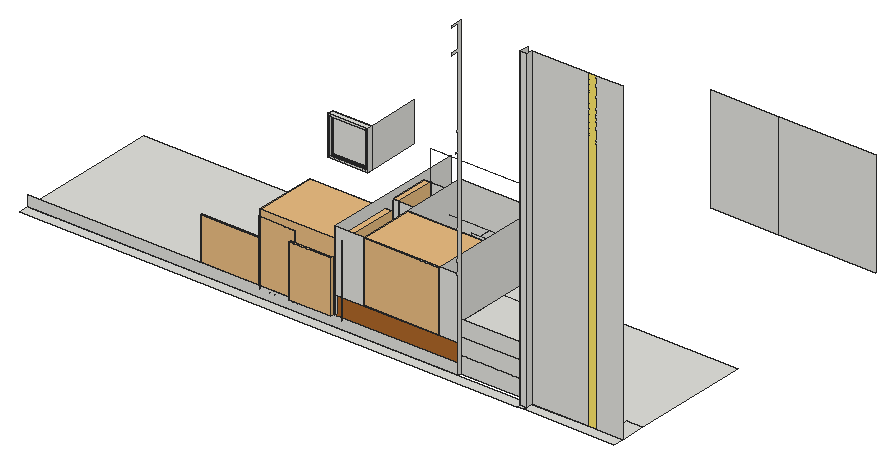
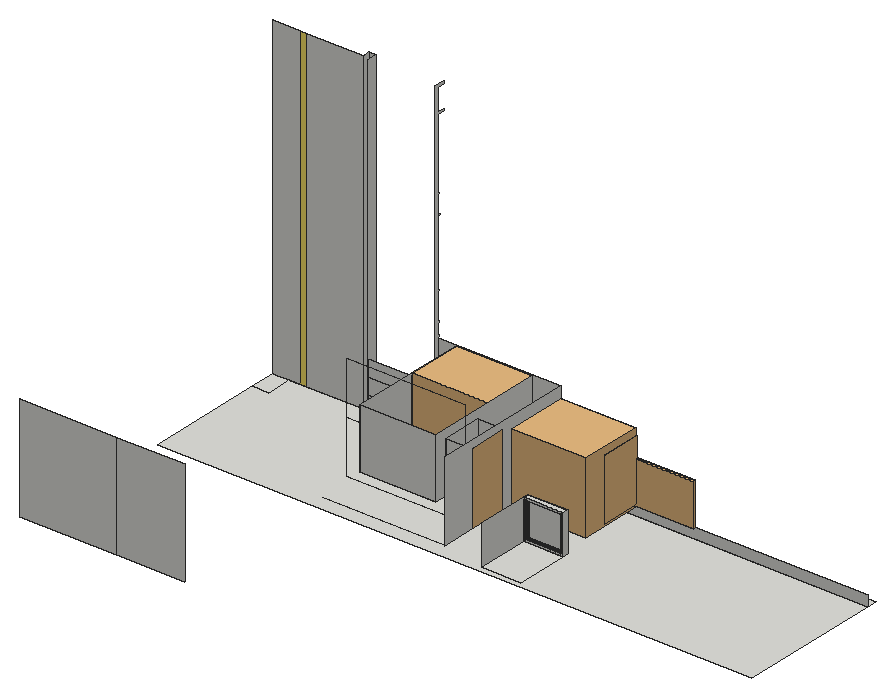
# SketchUp Ruby script. Lengths in inches.
U = 1.inch
M = Sketchup.active_model
def pt(a) = Geom::Point3d.new(a.map { |v| v * U })
def face(e, loops, mat)
  f = e.add_face(loops[0].map { |a| pt(a) })
  loops[1..].each { |l| e.add_face(l.map { |a| pt(a) }).erase! }
  f.material = f.back_material = mat if mat
  f
end
# faces: each face lists its corners as indices into pts; further lists are holes
def faces(e, pts, list, mat = nil) = list.each { |f| face(e, (f[0].is_a?(Array) ? f : [f]).map { |l| l.map { |i| pts[i] } }, mat) }
# xy, xz, yz: faces in a plane at the given z, y or x. An outline is a flat list of corners, or four numbers for a rectangle; further outlines are holes
def ring(l) = l.size == 4 ? [[l[0], l[1]], [l[2], l[1]], [l[2], l[3]], [l[0], l[3]]] : l.each_slice(2).to_a
def flat(e, list, mat, &to3) = list.each { |f| face(e, (f[0].is_a?(Array) ? f : [f]).map { |l| ring(l).map { |u, v| to3.(u, v) } }, mat) }
def xy(e, z, list, mat = nil) = flat(e, list, mat) { |x, y| [x, y, z] }
def xz(e, y, list, mat = nil) = flat(e, list, mat) { |x, z| [x, y, z] }
def yz(e, x, list, mat = nil) = flat(e, list, mat) { |y, z| [x, y, z] }
def lines(e, pts, list) = list.each { |a, b| e.add_line(pt(pts[a]), pt(pts[b])) }
# prism: a flat outline (further loops are holes) pulled along v
def prism(e, loops, v, mat = nil)
  f = face(e, loops, mat); d = Geom::Vector3d.new(v.map { |x| x * U })
  f.pushpull(f.normal.samedirection?(d) ? d.length : -d.length)
end
def box(e, o, s, mat = nil) = prism(e, [[o, [o[0] + s[0], o[1], o[2]], [o[0] + s[0], o[1] + s[1], o[2]], [o[0], o[1] + s[1], o[2]]]], [0, 0, s[2]], mat)
def at(x, y, z, deg = 0) = Geom::Transformation.translation(pt([x, y, z])) * Geom::Transformation.rotation(ORIGIN, Z_AXIS, deg.degrees)
def axes(o, x, y, z) = Geom::Transformation.new([*x, 0, *y, 0, *z, 0, *pt(o).to_a, 1])
def part(name) = M.definitions.add(name)
# library, detail: a bought-in or finely detailed component or shape, given as its bounding box
def library(name, o, s) = part(name).tap { |d| box(d.entities, o, s) }
def detail(e, o, s) = box(e.add_group.entities, o, s)
def put(e, d, t, mat = nil) = e.add_instance(d, t).tap { |i| i.material = mat if mat }
def group(e, t, mat = nil) = e.add_group.tap { |g| g.transformation = t; g.material = mat if mat }.entities
root = M.entities
M.materials.add("Generic").color = [255, 233, 107]
M.materials.add("[Wood Bamboo]").color = [173, 103, 41]
c1 = part("Copyright 2018, ")
xy(c1.entities,0.05,[[[19.06,0,19.06,9.82,21.3125,9.82,22.13,9.76,22.85,9.6,23.48,9.33,24,8.95,24.43,8.48,24.73,7.92,24.91,7.28,24.97,6.54,24.91,5.85,24.74,5.21,24.46,4.64,24.0625,4.14,23.58,3.73,23.03,3.4375,22.42,3.26,21.75,3.2,21.1,3.27,20.375,3.48,20.375,0],[21.62,4.3125,22.05,4.35,22.4375,4.47,22.79,4.66,23.09,4.94,23.34,5.28,23.52,5.66,23.63,6.09,23.67,6.56,23.6,7.16,23.4,7.68,23.08,8.1,22.66,8.39,22.08,8.56,21.28,8.61,20.375,8.61,20.375,4.61,20.98,4.39]],[25.77,0,27.98,4.71,25.47,9.82,26.9375,9.82,28.69,6.14,30.375,9.82,31.82,9.82,27.21,0],[[43.77,0,43.11,0.03,42.52,0.14,41.99,0.3125,41.54,0.55,41.18,0.86,40.92,1.2,40.77,1.6,40.71,2.04,40.82,2.64,41.12,3.13,41.63,3.5,42.35,3.75,41.86,4.16,41.74,4.37,41.7,4.57,41.77,4.87,41.98,5.14,42.3,5.36,42.73,5.51,42.1,5.88,41.65,6.34,41.38,6.91,41.29,7.57,41.34,8.0625,41.48,8.5,41.72,8.88,42.05,9.21,42.47,9.48,42.95,9.67,43.5,9.78,44.13,9.82,46.81,9.82,46.81,8.8125,45.49,8.8125,46.02,8.11,46.13,7.77,46.17,7.38,46.1,6.875,45.88,6.38,45.55,5.94,45.13,5.625,44.53,5.39,43.64,5.21,43.09,5.03,42.96,4.89,42.91,4.71,42.98,4.5,43.18,4.34,44.17,4.04,45.71,3.625,46.33,3.2,46.67,2.67,46.79,2.03,46.74,1.59,46.59,1.2,46.33,0.85,45.97,0.55,45.52,0.31,45.01,0.14,44.42,0.03],[43.74,1.02,44.5,1.09,45.0625,1.28,45.42,1.58,45.53,1.99,45.5,2.2,45.39,2.4,44.94,2.72,44.26,2.9375,43.41,3.01,42.82,2.94,42.34,2.73,42.03,2.42,41.93,2.03,42.04,1.59,42.38,1.28,42.95,1.09],[43.72,6.34,44.22,6.42,44.63,6.67,44.91,7.05,45,7.51,44.9,7.98,44.63,8.36,44.22,8.61,43.71,8.7,43.23,8.61,42.82,8.35,42.54,7.96,42.45,7.5,42.54,7.04,42.8125,6.67,43.22,6.42]],[180.16,0,182.36,4.71,179.85,9.82,181.32,9.82,183.07,6.14,184.75,9.82,186.2,9.82,181.59,0],[[219.8,0,219.13,0.03,218.54,0.14,218.02,0.3125,217.57,0.55,217.21,0.86,216.95,1.2,216.79,1.6,216.74,2.04,216.84,2.64,217.15,3.13,217.66,3.5,218.375,3.75,217.89,4.16,217.77,4.37,217.72,4.57,217.79,4.87,218,5.14,218.33,5.36,218.76,5.51,218.13,5.88,217.68,6.34,217.41,6.91,217.32,7.57,217.37,8.0625,217.51,8.5,217.75,8.88,218.08,9.21,218.5,9.48,218.98,9.67,219.53,9.78,220.16,9.82,222.83,9.82,222.83,8.8125,221.52,8.8125,222.05,8.11,222.16,7.77,222.2,7.38,222.125,6.875,221.91,6.38,221.58,5.94,221.16,5.625,220.5625,5.39,219.67,5.21,219.12,5.03,218.99,4.89,218.94,4.71,219.01,4.5,219.21,4.34,220.2,4.04,221.73,3.625,222.35,3.2,222.7,2.67,222.82,2.03,222.77,1.59,222.61,1.2,222.36,0.85,222,0.55,221.55,0.31,221.03,0.14,220.45,0.03],[219.77,1.02,220.53,1.09,221.09,1.28,221.44,1.58,221.5625,1.99,221.52,2.2,221.41,2.4,220.97,2.72,220.29,2.9375,219.43,3.01,218.84,2.94,218.37,2.73,218.0625,2.42,217.96,2.03,218.07,1.59,218.41,1.28,218.98,1.09],[219.75,6.34,220.25,6.42,220.66,6.67,220.93,7.05,221.02,7.51,220.93,7.98,220.66,8.36,220.24,8.61,219.74,8.7,219.25,8.61,218.85,8.35,218.57,7.96,218.48,7.5,218.57,7.04,218.84,6.67,219.25,6.42]],
  [92.62,1.6,92.62,1.87,92.89,2.17,93.07,2.48,93.22,3.3125,92.89,3.45,92.65,3.66,92.51,3.92,92.47,4.24,92.53,4.6,92.72,4.9,93.01,5.11,93.34,5.18,93.73,5.08,94.04,4.8,94.25,4.36,94.32,3.82,94.2,3.09,93.87,2.45,93.33,1.9375],[6.01,3.2,5.21,3.24,4.48,3.37,3.81,3.58,3.2,3.87,2.66,4.23,2.17,4.66,1.74,5.14,1.38,5.7,1.08,6.29,0.875,6.91,0.75,7.55,0.71,8.22,0.8,9.25,1.09,10.2,1.57,11.07,2.24,11.84,3.06,12.49,3.96,12.95,4.95,13.22,6.04,13.3125,6.83,13.26,7.68,13.11,8.5625,12.86,9.49,12.5,9.49,10.98,8.63,11.42,7.78,11.72,6.9375,11.91,6.11,11.97,5.29,11.9,4.55,11.7,3.89,11.37,3.29,10.9,2.8,10.33,2.45,9.7,2.24,8.99,2.17,8.22,2.24,7.44,2.45,6.74,2.79,6.11,3.27,5.55,3.86,5.09,4.53,4.76,5.27,4.57,6.09,4.5,6.98,4.57,7.87,4.78,8.74,5.12,9.6,5.6,9.6,4.05,8.79,3.68,7.92,3.41,6.99,3.25],[[14.21,3.2,13.51,3.26,12.87,3.4375,12.29,3.73,11.77,4.14,11.34,4.65,11.03,5.21,10.85,5.82,10.78,6.5,10.85,7.1875,11.03,7.81,11.34,8.375,11.78,8.88,12.31,9.3,12.9,9.59,13.55,9.77,14.27,9.83,14.98,9.77,15.63,9.59,16.21,9.29,16.73,8.87,17.16,8.36,17.47,7.79,17.66,7.16,17.72,6.47,17.66,5.79,17.47,5.18,17.16,4.625,16.72,4.13,16.19,3.72,15.6,3.43,14.9375,3.26],[14.25,4.4,14.71,4.44,15.12,4.55,15.48,4.74,15.81,5,16.07,5.32,16.26,5.68,16.37,6.08,16.41,6.53,16.37,6.97,16.25,7.375,16.06,7.74,15.78,8.0625,15.45,8.33,15.07,8.52,14.65,8.63,14.2,8.67,13.76,8.63,13.36,8.52,13,8.33,12.68,8.0625,12.42,7.74,12.23,7.37,12.12,6.97,12.08,6.52,12.12,6.07,12.24,5.67,12.43,5.31,12.69,4.99,13.02,4.73,13.39,4.55,13.8,4.44]],[57.3125,3.2,56.51,3.33,55.84,3.72,55.54,4.07,55.34,4.58,55.26,5.77,55.26,8.66,54.13,8.66,54.13,8.78,56.54,11.16,56.54,9.82,58.6,9.82,58.6,8.66,56.54,8.66,56.54,5.48,56.6,4.99,56.78,4.64,57.06,4.43,57.47,4.36,58.18,4.48,58.93,4.82,58.93,3.62,58.16,3.31],[[88.3125,3.2,87.67,3.25,87.08,3.41,86.54,3.66,86.06,4.02,85.66,4.45,85.37,4.93,85.2,5.46,85.14,6.04,85.23,6.75,85.49,7.37,85.93,7.91,86.54,8.36,86,8.86,85.64,9.37,85.4375,9.91,85.37,10.54,85.43,11.1,85.59,11.61,85.86,12.08,86.24,12.51,86.7,12.86,87.21,13.11,87.76,13.26,88.37,13.3125,88.96,13.26,89.51,13.11,90.01,12.86,90.46,12.51,90.83,12.09,91.09,11.62,91.25,11.1,91.31,10.54,91.23,9.91,91,9.33,90.62,8.82,90.08,8.36,90.68,7.91,91.11,7.38,91.36,6.75,91.45,6.02,91.39,5.4375,91.23,4.91,90.95,4.43,90.56,4,90.08,3.65,89.55,3.4,88.96,3.25],[88.33,4.54,89,4.64,89.54,4.94,89.9,5.39,90.02,5.96,90.02,6.11,89.9,6.72,89.54,7.21,88.98,7.53,88.28,7.64,87.6,7.53,87.05,7.21,86.69,6.71,86.57,6.09,86.69,5.47,87.06,4.98,87.62,4.65],[88.35,9.02,88.95,9.125,89.45,9.45,89.79,9.93,89.9,10.49,89.79,11.08,89.46,11.55,88.96,11.87,88.34,11.97,87.72,11.87,87.22,11.5625,86.89,11.09,86.78,10.51,86.89,9.9375,87.24,9.46,87.75,9.13]],
  [[113.29,3.2,112.92,3.24,112.64,3.36,112.43,3.57,112.32,3.85,111.9,3.57,111.47,3.375,111.03,3.26,110.57,3.22,109.95,3.33,109.44,3.66,109.1,4.17,108.99,4.79,109.1,5.375,109.43,5.89,109.97,6.32,110.6875,6.66,112.33,7.22,112.33,7.57,112.26,8.08,112.04,8.45,111.67,8.67,111.16,8.74,110.64,8.67,110.12,8.47,109.61,8.13,109.11,7.65,109.11,9.06,109.53,9.45,110.02,9.72,110.6,9.89,111.27,9.94,111.77,9.91,112.21,9.81,112.61,9.63,112.95,9.39,113.34,8.92,113.55,8.34,113.6,7.22,113.6,4.46,113.65,4.21,113.82,4.13,114.12,4.21,114.55,4.47,114.55,3.6875,113.85,3.3],[111.19,4.1,111.79,4.22,112.33,4.6,112.33,6.53,111.47,6.2,110.91,5.9375,110.54,5.67,110.34,5.375,110.27,5.01,110.33,4.64,110.53,4.35,110.82,4.16]],[121.02,3.2,120.43,3.28,119.88,3.51,119.43,3.87,119.1,4.34,118.9,5.04,118.83,6.09,118.83,9.82,120.12,9.82,120.12,6.11,120.19,5.24,120.41,4.68,120.82,4.38,121.44,4.28,121.88,4.33,122.29,4.5,122.66,4.78,123,5.17,123,9.82,124.29,9.82,124.29,3.3125,123,3.3125,123,4.15,122.5625,3.75,122.07,3.45,121.54,3.26],[[156.36,3.2,155.99,3.24,155.7,3.36,155.5,3.57,155.39,3.85,154.97,3.57,154.54,3.375,154.1,3.26,153.64,3.22,153.02,3.33,152.51,3.66,152.17,4.17,152.06,4.79,152.17,5.375,152.5,5.89,153.03,6.32,153.75,6.66,155.4,7.22,155.4,7.57,155.33,8.08,155.11,8.45,154.74,8.67,154.23,8.74,153.7,8.67,153.1875,8.47,152.68,8.13,152.18,7.65,152.18,9.06,152.59,9.45,153.09,9.72,153.67,9.89,154.33,9.94,154.83,9.91,155.28,9.81,155.68,9.63,156.02,9.39,156.4,8.92,156.62,8.34,156.66,7.22,156.66,4.46,156.72,4.21,156.89,4.13,157.1875,4.21,157.62,4.47,157.62,3.6875,156.92,3.3],[154.26,4.1,154.85,4.22,155.4,4.6,155.4,6.53,154.54,6.2,153.98,5.9375,153.61,5.67,153.4,5.375,153.34,5.01,153.4,4.64,153.59,4.35,153.89,4.16]],[161.74,3.2,161.01,3.26,160.37,3.43,159.8,3.71,159.3,4.11,158.91,4.6,158.62,5.16,158.45,5.81,158.4,6.53,158.45,7.26,158.62,7.92,158.89,8.5,159.28,9,159.76,9.41,160.3,9.71,160.92,9.88,161.6,9.94,162.51,9.85,163.49,9.49,163.49,8.12,162.55,8.59,161.68,8.74,161.27,8.7,160.89,8.59,160.55,8.4,160.25,8.13,160.01,7.8,159.84,7.4375,159.73,7.02,159.7,6.57,159.73,6.1,159.85,5.68,160.04,5.31,160.3,4.99,160.63,4.73,161.01,4.55,161.44,4.4375,161.93,4.4,162.73,4.51,163.63,4.83,163.63,3.5625,162.67,3.29],[[178.37,3.2,178,3.24,177.71,3.36,177.51,3.57,177.39,3.85,176.98,3.57,176.55,3.375,176.1,3.26,175.65,3.22,175.02,3.33,174.52,3.66,174.18,4.17,174.0625,4.79,174.17,5.375,174.51,5.89,175.04,6.32,175.76,6.66,177.41,7.22,177.41,7.57,177.33,8.08,177.11,8.45,176.75,8.67,176.23,8.74,175.71,8.67,175.19,8.47,174.6875,8.13,174.18,7.65,174.18,9.06,174.6,9.45,175.1,9.72,175.68,9.89,176.34,9.94,176.84,9.91,177.29,9.81,177.68,9.63,178.03,9.39,178.41,8.92,178.625,8.34,178.67,7.22,178.67,4.46,178.73,4.21,178.9,4.13,179.2,4.21,179.625,4.47,179.625,3.6875,178.92,3.3],[176.27,4.1,176.86,4.22,177.41,4.6,177.41,6.53,176.54,6.2,175.98,5.9375,175.61,5.67,175.41,5.375,175.34,5.01,175.41,4.64,175.6,4.35,175.9,4.16]],
  [210.76,3.2,209.73,3.33,208.59,3.78,208.59,5.17,209.71,4.55,210.23,4.37,210.66,4.3125,211.04,4.36,211.36,4.51,211.57,4.73,211.65,4.98,211.6,5.24,211.46,5.45,210.65,5.99,209.62,6.64,209.02,7.18,208.73,7.69,208.64,8.25,208.67,8.6,208.78,8.93,208.96,9.22,209.22,9.47,209.89,9.83,210.72,9.94,211.6875,9.81,212.68,9.41,212.68,8.13,211.64,8.65,210.81,8.83,210.47,8.79,210.2,8.67,210.03,8.48,209.97,8.25,210.02,8.03,210.18,7.82,210.91,7.32,211.37,7.06,212.08,6.59,212.59,6.09,212.89,5.57,213,5.02,212.96,4.64,212.84,4.3,212.64,3.99,212.37,3.71,212.04,3.49,211.66,3.33],[[73.82,3.22,73.14,3.3,72.53,3.56,71.99,3.99,71.52,4.59,71.14,5.34,70.87,6.2,70.7,7.17,70.65,8.25,70.71,9.32,70.875,10.29,71.16,11.15,71.55,11.9,72.03,12.52,72.58,12.96,73.2,13.23,73.88,13.3125,74.53,13.23,75.12,12.96,75.65,12.51,76.125,11.89,76.51,11.13,76.79,10.27,76.96,9.32,77.01,8.28,76.96,7.2,76.79,6.24,76.51,5.38,76.125,4.62,75.65,4.01,75.11,3.57,74.5,3.3],[73.81,4.52,74.2,4.58,74.54,4.77,74.84,5.08,75.1,5.51,75.31,6.06,75.46,6.6875,75.58,8.22,75.46,9.76,75.32,10.4,75.12,10.95,74.87,11.4,74.59,11.72,74.26,11.91,73.89,11.97,73.82,11.97,73.4375,11.91,73.09,11.72,72.79,11.41,72.53,10.97,72.32,10.43,72.18,9.79,72.06,8.26,72.17,6.7,72.32,6.06,72.52,5.51,72.78,5.08,73.08,4.77,73.42,4.58]],[[204.86,3.22,203.89,3.33,203.125,3.66,202.53,4.18,202.06,4.86,201.76,5.67,201.66,6.6,201.71,7.31,201.87,7.95,202.13,8.51,202.5,9.01,202.95,9.42,203.47,9.71,204.05,9.89,204.6875,9.94,205.3,9.89,205.85,9.72,206.33,9.43,206.75,9.04,207.09,8.55,207.33,7.98,207.47,7.34,207.52,6.61,207.52,6.45,202.95,6.45,203.13,5.61,203.32,5.27,203.57,4.97,203.88,4.73,204.23,4.55,205.06,4.42,205.68,4.47,206.28,4.61,206.86,4.86,207.41,5.21,207.41,3.95,206.82,3.61,206.23,3.39,205.6,3.26],[202.98,7.22,206.25,7.22,206.11,7.9,205.79,8.41,205.31,8.72,204.6875,8.83,204.06,8.72,203.55,8.41,203.1875,7.9]],[32.81,3.3125,32.81,9.82,34.1,9.82,34.1,8.33,34.17,8.4375,34.64,9.1,35.1,9.57,35.57,9.85,36.04,9.94,36.4,9.9,36.78,9.76,37.55,9.21,36.875,8.08,36.23,8.55,35.63,8.71,35.33,8.68,35.05,8.57,34.55,8.12,34.21,7.47,34.1,6.71,34.1,3.3125],[38.48,3.3125,39.77,9.82],
  [47.77,3.3125,47.77,13.1875,49.06,13.1875,49.06,8.96,49.49,9.39,49.96,9.7,50.49,9.88,51.06,9.94,51.68,9.86,52.23,9.62,52.68,9.23,52.99,8.72,53.18,8.01,53.24,7.02,53.24,3.3125,51.96,3.3125,51.96,7.34,51.87,7.98,51.61,8.48,51.2,8.81,50.6875,8.92,50.27,8.86,49.89,8.7,49.49,8.41,49.06,7.97,49.06,3.3125],[63.46,3.3125,63.46,3.41,64.06,4.11,66.27,7.04,66.95,8.09,67.35,8.86,67.53,9.47,67.6,10.07,67.48,10.82,67.125,11.41,66.57,11.79,65.87,11.92,65.28,11.83,64.7,11.57,64.15,11.14,63.66,10.58,63.66,12.375,64.24,12.79,64.83,13.08,65.43,13.26,66.04,13.3125,66.65,13.26,67.21,13.1,67.72,12.83,68.17,12.45,68.53,11.99,68.79,11.47,68.95,10.9,69,10.26,68.95,9.65,68.8,8.99,68.51,8.27,68.06,7.4375,67.34,6.4,66.26,5.04,65.95,4.68,69.71,4.68,69.71,3.3125],[80.37,3.3125,81.78,13.1875],[100.21,3.3125,100.21,13.1875,101.625,13.1875,101.625,8.67,105.78,13.1875,107.55,13.1875,103.27,8.5,108.6,3.3125,106.67,3.3125,101.625,8.19,101.625,3.3125],[115.72,3.3125,117,13.1875],
  [126.04,3.3125,126.04,9.82,127.33,9.82,127.33,8.96,127.82,9.39,128.3,9.7,128.78,9.88,129.25,9.94,129.83,9.87,130.35,9.65,130.79,9.28,131.17,8.77,131.6875,9.29,132.22,9.66,132.77,9.88,133.32,9.96,133.77,9.91,134.18,9.78,134.55,9.57,134.88,9.27,135.15,8.875,135.34,8.39,135.45,7.82,135.49,7.15,135.49,3.3125,134.2,3.3125,134.2,7.17,134.12,7.88,133.87,8.41,133.47,8.73,132.92,8.84,132.53,8.79,132.15,8.64,131.78,8.39,131.43,8.04,131.43,3.3125,130.13,3.3125,130.13,6.93,130.0625,7.85,129.84,8.44,129.67,8.63,129.45,8.76,128.83,8.87,128.45,8.82,128.1,8.6875,127.74,8.43,127.33,8.04,127.33,3.3125],[141.43,3.3125,141.43,13.1875,142.77,13.1875,146.05,9.13,149.31,13.1875,150.63,13.1875,150.63,3.3125,149.21,3.3125,149.21,11,146.17,7.18,145.91,7.18,142.84,11,142.84,3.3125],[165.29,3.3125,165.29,13.1875,166.7,13.1875,166.7,8.67,170.86,13.1875,172.62,13.1875,168.34,8.5,173.67,3.3125,171.75,3.3125,166.7,8.19,166.7,3.3125],[214.51,3.3125,215.8,9.82],[223.8,3.3125,223.8,9.82,225.12,9.82,225.12,8.99,225.5625,9.41,226.04,9.7,226.54,9.88,227.07,9.94,227.66,9.86,228.2,9.63,228.67,9.26,229,8.77,229.2,8.06,229.27,7.03,229.27,3.3125,227.99,3.3125,227.99,7.02,227.91,7.87,227.68,8.44,227.28,8.76,226.66,8.87,226.23,8.8125,225.82,8.64,225.45,8.36,225.12,7.96,225.12,3.3125],
  [[191.3125,3.33,191.3125,13.1875,194.64,13.1875,195.6,13.15,196.45,13.04,197.19,12.85,197.83,12.58,198.39,12.25,198.88,11.84,199.32,11.36,199.7,10.81,200,10.21,200.22,9.58,200.35,8.93,200.39,8.25,200.29,7.28,200.01,6.35,199.54,5.5,198.92,4.76,198.14,4.14,197.24,3.7,196.22,3.4,194.4375,3.33],[192.73,4.59,194.54,4.59,195.48,4.62,196.18,4.73,197.16,5.1,197.88,5.65,198.34,6.21,198.66,6.85,198.86,7.55,198.93,8.33,198.86,9.08,198.66,9.77,198.32,10.38,197.85,10.92,197.43,11.26,196.94,11.53,195.97,11.85,194.49,11.93,192.73,11.93]],[39.12,11.03,38.84,11.09,38.59,11.26,38.42,11.51,38.37,11.8,38.42,12.08,38.59,12.32,38.84,12.49,39.12,12.55,39.41,12.5,39.66,12.33,39.83,12.09,39.89,11.8,39.83,11.51,39.66,11.26,39.41,11.09],[215.14,11.03,214.87,11.09,214.62,11.26,214.45,11.51,214.4,11.8,214.45,12.08,214.62,12.32,214.87,12.49,215.14,12.55,215.44,12.5,215.6875,12.33,215.86,12.09,215.92,11.8,215.86,11.51,215.6875,11.26,215.44,11.09]])
c2 = library("Glass Railings(black Handrails)",[-57.04,-132.55,0],[169.29,2.52,28.17])
c3 = library("cay+chuoi",[26.89,19.66,0.52],[41.96,45.65,69.71])
c4 = library("Rectangular Planter with Plant",[-49.93,-33.04,0],[93.24,71.01,81.08])
c5 = library("KentiaPalm",[-22.86,-14.31,0],[47.49,43.96,59.125])
c6 = library("Untitled (14)",[0,0,0],[7.13,36,83])
c7 = library("Group\#14",[0,0,0],[39.5,117.4375,51.17])
c8 = part("Group668\#1")
p = [[0,0,0],[0,0,-13.34],[-3.03,0,-13.34],[19.7,-23.5,0],[-19.7,-23.5,0],[19.7,23.5,0],
  [19.7,0,0],[-19.7,23.5,0],[3.03,0,-13.34],[-19.7,0,0],[0,0,-21.6]]
lines(c8.entities,p,[[0,1],[1,2],[3,4],[5,6],[7,5],[1,8],[9,0],[0,6],[8,10],[4,9],[6,3],[2,10],
  [9,7]])
c9 = part("Rectangle Light")
put(c9.entities,c8,at(0,0,0))
xy(root,112.51,[[624.25,904.1875,1189.1875,916.1875],[1189.1875,904.1875,1197.1875,908.4375],[1197.1875,904.1875,1299.8125,916.1875],[1189.1875,908.4375,1197.1875,916.1875],[624.25,916.1875,624.25,1080.1875,1299.8125,1080.1875,1299.8125,945.21,1281.875,945.21,1281.875,916.1875,1189.1875,916.1875,1189.1875,919.75,1112.75,919.75,1112.75,916.1875],
  [1281.875,916.1875,1299.8125,945.21]])
xy(root,145.85,[[1005.21,916.1875,1091.46,1053.125]])
xy(root,164.6,[[834.07,1080.1875,878.82,1086.1875],[834.07,1080.1875,878.82,1146.3125]])
xy(root,166.76,[[836.23,1080.1875,876.66,1081.4375],[836.23,1084.9375,876.66,1086.1875]])
xy(root,167.39,[[836.87,1081.4375,876.02,1082.6875],[836.87,1082.6875,876.02,1083.6875],[836.87,1083.6875,876.02,1084.9375]])
xy(root,167.92,[[837.4,1082.6875,875.5,1082.79],[837.4,1082.79,875.5,1083.59],[837.4,1083.59,875.5,1083.6875]])
xy(root,206.03,[[837.4,1082.6875,875.5,1082.79],[837.4,1082.79,875.5,1083.59],[837.4,1083.59,875.5,1083.6875]])
xy(root,206.55,[[836.87,1081.4375,876.02,1082.6875],[836.87,1082.6875,876.02,1083.6875],[836.87,1083.6875,876.02,1084.9375]])
xy(root,207.1875,[[836.23,1080.1875,876.66,1081.4375],[836.23,1084.9375,876.66,1086.1875]])
xy(root,209.35,[[834.07,1080.1875,878.82,1086.1875]])
xz(root,908.4375,[[1189.1875,112.51,1197.1875,472.51]])
xz(root,916.1875,[[624.25,112.51,1112.75,112.51,1112.75,124.53,975.58,124.53,975.58,144.9,973.0625,144.9,973.0625,124.51,624.25,124.51],[1197.1875,112.51,1261.34,472.51],[1269.34,112.51,1299.8125,472.51],[[973.0625,144.9,1112.75,215.04],[1005.21,145.85,1091.46,214.23]]])
xz(root,916.1875,[[1261.34,112.51,1269.34,472.51]],"Generic")
xz(root,916.1875,[[975.58,124.53,1112.75,144.9]],"[Wood Bamboo]")
xz(root,919.75,[[1112.75,112.51,1189.1875,131.11],[1112.75,131.11,1189.1875,149.71],[1112.75,149.71,1189.1875,168.31]])
xz(root,998.1875,[[973.0625,124.51,1001.875,206.83]])
xz(root,1042.875,[[973.0625,124.51,1001.875,206.83]])
xz(root,1053.125,[[1005.21,145.85,1091.46,214.23]])
xz(root,1080.1875,[[[834.07,164.6,878.82,209.35],[836.23,166.76,876.66,207.1875]]])
xz(root,1081.4375,[[[836.23,166.76,876.66,207.1875],[836.87,167.39,876.02,206.55]]])
xz(root,1082.6875,[[[836.87,167.39,876.02,206.55],[837.4,167.92,875.5,206.03]]])
xz(root,1082.79,[[837.4,167.92,875.5,206.03]])
xz(root,1083.59,[[837.4,167.92,875.5,206.03]])
xz(root,1083.6875,[[[836.87,167.39,876.02,206.55],[837.4,167.92,875.5,206.03]]])
xz(root,1084.9375,[[[836.23,166.76,876.66,207.1875],[836.87,167.39,876.02,206.55]]])
xz(root,1086.1875,[[[834.07,164.6,878.82,209.35],[836.23,166.76,876.66,207.1875]]])
xz(root,1276.1875,[[1112.75,124.51,1189.1875,244.51],[1189.1875,124.51,1299.8125,244.51]])
yz(root,834.07,[[1080.1875,164.6,1086.1875,209.35]])
yz(root,836.23,[[1080.1875,166.76,1081.4375,207.1875],[1084.9375,166.76,1086.1875,207.1875]])
yz(root,836.87,[[1081.4375,167.39,1082.6875,206.55],[1082.6875,167.39,1083.6875,206.55],[1083.6875,167.39,1084.9375,206.55]])
yz(root,837.4,[[1082.6875,167.92,1082.79,206.03],[1082.79,167.92,1083.59,206.03],[1083.59,167.92,1083.6875,206.03]])
yz(root,875.5,[[1082.6875,167.92,1082.79,206.03],[1082.79,167.92,1083.59,206.03],[1083.59,167.92,1083.6875,206.03]])
yz(root,876.02,[[1081.4375,167.39,1082.6875,206.55],[1082.6875,167.39,1083.6875,206.55],[1083.6875,167.39,1084.9375,206.55]])
yz(root,876.66,[[1080.1875,166.76,1081.4375,207.1875],[1084.9375,166.76,1086.1875,207.1875]])
yz(root,878.82,[[1080.1875,164.6,1086.1875,209.35],[1080.1875,164.6,1146.3125,209.35]])
yz(root,973.0625,[[916.1875,124.51,916.1875,215.04,1080.1875,215.04,1080.1875,124.51,1042.875,124.51,1042.875,206.83,998.1875,206.83,998.1875,124.51]])
yz(root,1001.875,[[998.1875,124.51,1042.875,206.83]])
yz(root,1005.21,[[916.1875,145.85,1053.125,214.23]])
yz(root,1091.46,[[916.1875,145.85,1053.125,214.23]])
yz(root,1112.75,[[916.1875,112.51,919.75,112.51,919.75,472.51,907.15,472.51,907.15,469.7,916.1875,469.7,916.1875,444.51,907.15,444.51,907.15,441.7,916.1875,441.7,916.1875,361.64,915.15,361.64,915.15,360.64,916.1875,360.64,916.1875,340.08,913.52,340.08,913.52,339.08,916.1875,339.08,916.1875,262.47,914.15,262.47,914.15,261.47,916.1875,261.47,916.1875,230.78,914.15,230.78,914.15,228.78,916.1875,228.78,916.1875,217.04,914.15,217.04,914.15,215.04,916.1875,215.04]])
yz(root,1189.1875,[[908.4375,112.51,919.75,472.51]])
yz(root,1197.1875,[[908.4375,112.51,916.1875,472.51]])
p = [[973.0625,1080.1875,124.51],[1112.75,1080.1875,124.51],[973.29,916.1875,144.9],[973.29,917.03,125.38]]
lines(root,p,[[0,1],[2,3]])
put(root,c1,axes([840.86,1084.41,164.6],[0.13928,0,0],[0,-0.1494,0],[0,0,-0.93236]))
put(root,c2,axes([871.68,1048.73,124.51],[0.90532,0,0],[0,1,0],[0,0,1.70393]))
put(root,c3,at(859,896.52,124.53))
put(root,c4,at(937.65,949.23,121.41))
put(root,c5,at(945.64,928.05,123.66))
put(root,c6,axes([973.0625,998.1875,124.51],[1,0,0],[0,1.24132,0],[0,0,0.99172]))
put(root,c7,axes([1005.38,916.1875,145.85],[2.1792,0,0],[0,0.536,0],[0,0,1.33625]))
put(root,c9,axes([1051.5,1037.49,184.88],[3.4393,0,0],[0,0,-2.56],[0,1,0]))
